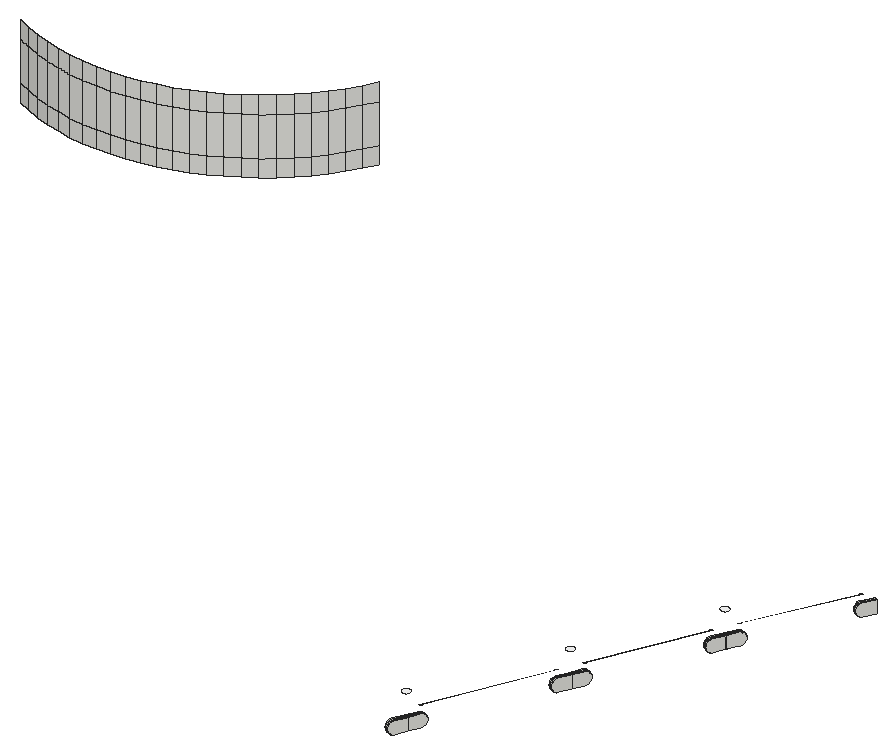
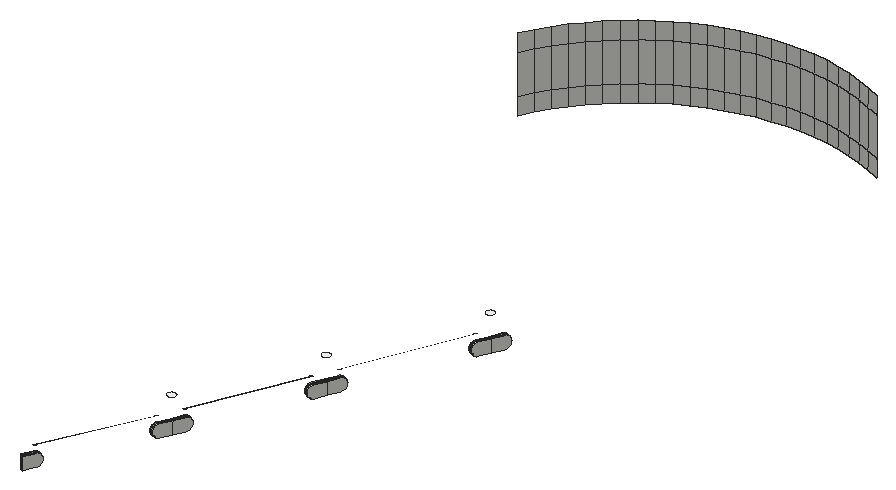
# SketchUp Ruby script. Lengths in inches.
U = 1.inch
M = Sketchup.active_model
def pt(a) = Geom::Point3d.new(a.map { |v| v * U })
def face(e, loops, mat)
  f = e.add_face(loops[0].map { |a| pt(a) })
  loops[1..].each { |l| e.add_face(l.map { |a| pt(a) }).erase! }
  f.material = f.back_material = mat if mat
  f
end
# faces: each face lists its corners as indices into pts; further lists are holes
def faces(e, pts, list, mat = nil) = list.each { |f| face(e, (f[0].is_a?(Array) ? f : [f]).map { |l| l.map { |i| pts[i] } }, mat) }
# xy, xz, yz: faces in a plane at the given z, y or x. An outline is a flat list of corners, or four numbers for a rectangle; further outlines are holes
def ring(l) = l.size == 4 ? [[l[0], l[1]], [l[2], l[1]], [l[2], l[3]], [l[0], l[3]]] : l.each_slice(2).to_a
def flat(e, list, mat, &to3) = list.each { |f| face(e, (f[0].is_a?(Array) ? f : [f]).map { |l| ring(l).map { |u, v| to3.(u, v) } }, mat) }
def xy(e, z, list, mat = nil) = flat(e, list, mat) { |x, y| [x, y, z] }
def xz(e, y, list, mat = nil) = flat(e, list, mat) { |x, z| [x, y, z] }
def yz(e, x, list, mat = nil) = flat(e, list, mat) { |y, z| [x, y, z] }
def lines(e, pts, list) = list.each { |a, b| e.add_line(pt(pts[a]), pt(pts[b])) }
# prism: a flat outline (further loops are holes) pulled along v
def prism(e, loops, v, mat = nil)
  f = face(e, loops, mat); d = Geom::Vector3d.new(v.map { |x| x * U })
  f.pushpull(f.normal.samedirection?(d) ? d.length : -d.length)
end
def box(e, o, s, mat = nil) = prism(e, [[o, [o[0] + s[0], o[1], o[2]], [o[0] + s[0], o[1] + s[1], o[2]], [o[0], o[1] + s[1], o[2]]]], [0, 0, s[2]], mat)
def at(x, y, z, deg = 0) = Geom::Transformation.translation(pt([x, y, z])) * Geom::Transformation.rotation(ORIGIN, Z_AXIS, deg.degrees)
def axes(o, x, y, z) = Geom::Transformation.new([*x, 0, *y, 0, *z, 0, *pt(o).to_a, 1])
def part(name) = M.definitions.add(name)
# library, detail: a bought-in or finely detailed component or shape, given as its bounding box
def library(name, o, s) = part(name).tap { |d| box(d.entities, o, s) }
def detail(e, o, s) = box(e.add_group.entities, o, s)
def put(e, d, t, mat = nil) = e.add_instance(d, t).tap { |i| i.material = mat if mat }
def group(e, t, mat = nil) = e.add_group.tap { |g| g.transformation = t; g.material = mat if mat }.entities
root = M.entities
M.materials.add("Glass_Safety_01").color = [204, 235, 244]
M.materials["Glass_Safety_01"].alpha = 0.1
M.materials.add("[Color_000]").color = [255, 255, 255]
xy(root,351.283,[[925.57,724.044,925.318,724.154,925.385,724.307,926.104,725.958,926.356,725.848],[925.137,724.232,924.884,724.342,925.67,726.147,925.923,726.037,925.204,724.386],[926.356,725.848,926.104,725.958,926.89,727.763,927.142,727.653],[925.923,726.037,925.67,726.147,926.456,727.952,926.709,727.842],[935.495,746.832,935.243,746.942,935.305,747.085,936.029,748.747,936.281,748.637],
  [935.062,747.021,934.809,747.131,935.595,748.935,935.848,748.825,935.124,747.164],[936.281,748.637,936.029,748.747,936.821,750.548,937.073,750.4375],[935.848,748.825,935.595,748.935,936.388,750.739,936.641,750.628],[944.885,768.202,944.633,768.313,944.699,768.465,945.424,770.112,945.673,769.993],[944.452,768.392,944.2,768.503,944.993,770.305,945.245,770.194,944.519,768.544],
  [945.673,769.993,945.424,770.112,945.425,770.115,945.677,770.004,945.675,769.999],[945.677,770.004,945.425,770.115,946.271,771.889,946.52,771.77],[945.246,770.197,944.997,770.315,945.844,772.092,946.093,771.974],[954.439,788.385,954.19,788.504,954.265,788.661,955.037,790.281,955.286,790.162],[954.013,788.589,953.764,788.707,954.6,790.46,954.857,790.359,954.087,788.745]])
xy(root,351.362,[[925.475,724.515,925.294,724.593,925.923,726.037,926.104,725.958],[926.104,725.958,925.923,726.037,926.552,727.481,926.732,727.402],[935.4,747.303,935.219,747.382,935.848,748.825,935.938,748.786,936.029,748.747],[936.029,748.747,935.938,748.786,935.848,748.825,936.482,750.267,936.662,750.188],[944.791,768.673,944.611,768.752,945.245,770.194,945.335,770.154,945.424,770.112],
  [945.424,770.112,945.335,770.154,945.425,770.115,945.424,770.113],[945.425,770.115,945.335,770.154,945.246,770.197,945.924,771.618,946.101,771.534]],"Glass_Safety_01")
xy(root,353.33,[[925.475,724.515,926.104,725.958,925.923,726.037,925.294,724.593],[926.104,725.958,926.732,727.402,926.552,727.481,925.923,726.037],[935.4,747.303,936.029,748.747,935.938,748.786,935.848,748.825,935.219,747.382],[936.029,748.747,936.662,750.188,936.482,750.267,935.848,748.825,935.938,748.786],[944.791,768.673,945.424,770.112,945.335,770.154,945.245,770.194,944.611,768.752],
  [945.424,770.112,945.424,770.113,945.425,770.115,945.335,770.154],[945.425,770.115,946.101,771.534,945.924,771.618,945.246,770.197,945.335,770.154]],"Glass_Safety_01")
xy(root,353.409,[[925.57,724.044,926.356,725.848,926.104,725.958,925.385,724.307,925.318,724.154],[925.137,724.232,925.204,724.386,925.923,726.037,925.67,726.147,924.884,724.342],[926.356,725.848,927.142,727.653,926.89,727.763,926.104,725.958],[925.923,726.037,926.709,727.842,926.456,727.952,925.67,726.147],[935.495,746.832,936.281,748.637,936.029,748.747,935.305,747.085,935.243,746.942],
  [935.062,747.021,935.124,747.164,935.848,748.825,935.595,748.935,934.809,747.131],[936.281,748.637,937.073,750.4375,936.821,750.548,936.029,748.747],[935.848,748.825,936.641,750.628,936.388,750.739,935.595,748.935],[944.885,768.202,945.673,769.993,945.424,770.112,944.699,768.465,944.633,768.313],[944.452,768.392,944.519,768.544,945.245,770.194,944.993,770.305,944.2,768.503],
  [945.673,769.993,945.675,769.999,945.677,770.004,945.425,770.115,945.424,770.112],[945.677,770.004,946.52,771.77,946.271,771.889,945.425,770.115],[945.246,770.197,946.093,771.974,945.844,772.092,944.997,770.315],[954.439,788.385,955.286,790.162,955.037,790.281,954.265,788.661,954.19,788.504],[954.013,788.589,954.087,788.745,954.857,790.359,954.6,790.46,953.764,788.707]])
xy(root,354.511,[[926.89,727.763,935.124,747.164,926.709,727.842],[926.89,727.763,935.305,747.085,935.124,747.164],[936.821,750.548,944.519,768.544,936.641,750.628],[936.821,750.548,944.7,768.465,944.519,768.544],[946.271,771.889,954.087,788.745,946.093,771.974],
  [946.271,771.889,954.265,788.661,954.087,788.745]],"Glass_Safety_01")
xy(root,357.267,[[926.058,725.369,926.219,725.402,926.367,725.476,926.489,725.585,926.58,725.723,926.632,725.879,926.642,726.043,926.609,726.204,926.535,726.351,926.426,726.474,926.289,726.564,926.132,726.616,925.968,726.626,925.807,726.593,925.66,726.519,925.537,726.41,925.447,726.273,925.395,726.117,925.385,725.953,925.418,725.792,925.492,725.645,925.601,725.522,925.738,725.431,925.894,725.379],[935.983,748.158,936.145,748.191,936.292,748.264,936.415,748.374,936.505,748.511,936.557,748.667,936.567,748.831,936.534,748.992,936.46,749.139,936.351,749.262,936.214,749.353,936.058,749.405,935.893,749.414,935.732,749.381,935.585,749.308,935.462,749.198,935.372,749.061,935.32,748.905,935.31,748.741,935.343,748.58,935.417,748.433,935.526,748.31,935.663,748.219,935.819,748.167],[945.38,769.526,945.541,769.559,945.688,769.633,945.811,769.742,945.902,769.879,945.954,770.035,945.963,770.199,945.93,770.361,945.857,770.508,945.747,770.631,945.61,770.721,945.454,770.773,945.29,770.783,945.129,770.75,944.982,770.676,944.859,770.567,944.768,770.43,944.716,770.274,944.707,770.109,944.74,769.948,944.813,769.801,944.923,769.678,945.06,769.588,945.216,769.536]],"[Color_000]")
p = [[926.356,725.848,353.409],[925.57,724.044,353.409],[925.46,723.791,353.373],[925.358,723.556,353.267],[925.27,723.354,353.098],[925.203,723.2,352.877],
  [925.16,723.102,352.621],[925.146,723.069,352.346],[925.16,723.102,352.071],[925.203,723.2,351.814],[925.27,723.354,351.594],[925.358,723.556,351.425],
  [925.46,723.791,351.319],[925.57,724.044,351.283],[926.356,725.848,351.283],[925.318,724.154,353.409],[925.385,724.307,353.409],[925.385,724.307,351.283],
  [925.318,724.154,351.283],[925.208,723.901,351.319],[925.105,723.666,351.425],[925.017,723.464,351.594],[924.95,723.31,351.814],[924.908,723.212,352.071],
  [924.893,723.179,352.346],[924.908,723.212,352.621],[924.95,723.31,352.877],[925.017,723.464,353.098],[925.105,723.666,353.267],[925.208,723.901,353.373],
  [925.137,724.232,351.283],[925.204,724.386,351.283],[925.204,724.386,353.409],[925.137,724.232,353.409],[925.027,723.98,353.373],[924.925,723.745,353.267],
  [924.837,723.543,353.098],[924.77,723.388,352.877],[924.727,723.291,352.621],[924.713,723.258,352.346],[924.727,723.291,352.071],[924.77,723.388,351.814],
  [924.837,723.543,351.594],[924.925,723.745,351.425],[925.027,723.98,351.319],[924.884,724.342,353.409],[925.67,726.147,353.409],[925.67,726.147,351.283],
  [924.884,724.342,351.283],[924.775,724.09,351.319],[924.672,723.855,351.425],[924.584,723.653,351.594],[924.517,723.498,351.814],[924.474,723.401,352.071],
  [924.46,723.368,352.346],[924.474,723.401,352.621],[924.517,723.498,352.877],[924.584,723.653,353.098],[924.672,723.855,353.267],[924.775,724.09,353.373],
  [926.104,725.958,351.283],[926.104,725.958,353.409],[926.104,725.958,353.33],[925.475,724.515,353.33],[925.475,724.515,351.362],[926.104,725.958,351.362],
  [925.923,726.037,353.409],[925.923,726.037,351.283],[925.923,726.037,351.362],[925.294,724.593,351.362],[925.294,724.593,353.33],[925.923,726.037,353.33],
  [927.142,727.653,353.409],[927.142,727.653,351.283],[927.252,727.905,351.319],[927.355,728.14,351.425],[927.442,728.342,351.594],[927.51,728.497,351.814],
  [927.552,728.594,352.071],[927.567,728.628,352.346],[927.552,728.594,352.621],[927.51,728.497,352.877],[927.442,728.342,353.098],[927.355,728.14,353.267],
  [927.252,727.905,353.373],[926.709,727.842,351.283],[926.709,727.842,353.409],[926.552,727.481,353.33],[926.552,727.481,351.362],[926.89,727.763,353.409],
  [926.89,727.763,351.283],[926.732,727.402,351.362],[926.732,727.402,353.33],[926.456,727.952,353.409],[926.566,728.204,353.373],[926.669,728.439,353.267],
  [926.757,728.641,353.098],[926.824,728.796,352.877],[926.866,728.893,352.621],[926.881,728.926,352.346],[926.866,728.893,352.071],[926.824,728.796,351.814],
  [926.757,728.641,351.594],[926.669,728.439,351.425],[926.566,728.204,351.319],[926.456,727.952,351.283],[926.999,728.015,351.319],[926.819,728.094,351.319],
  [926.819,728.094,353.373],[926.921,728.329,353.267],[927.009,728.531,353.098],[927.077,728.686,352.877],[927.119,728.783,352.621],[927.134,728.816,352.346],
  [927.119,728.783,352.071],[927.077,728.686,351.814],[927.009,728.531,351.594],[926.921,728.329,351.425],[927.102,728.25,351.425],[927.19,728.452,351.594],
  [927.257,728.607,351.814],[927.3,728.705,352.071],[927.314,728.738,352.346],[927.3,728.705,352.621],[927.257,728.607,352.877],[927.19,728.452,353.098],
  [927.102,728.25,353.267],[926.999,728.015,353.373],[936.281,748.637,353.409],[935.495,746.832,353.409],[935.385,746.58,353.373],[935.283,746.345,353.267],
  [935.195,746.143,353.098],[935.128,745.988,352.877],[935.085,745.891,352.621],[935.071,745.857,352.346],[935.085,745.891,352.071],[935.128,745.988,351.814],
  [935.195,746.143,351.594],[935.283,746.345,351.425],[935.385,746.58,351.319],[935.495,746.832,351.283],[936.281,748.637,351.283],[935.062,747.021,351.283],
  [935.124,747.164,351.283],[935.124,747.164,353.409],[935.062,747.021,353.409],[934.952,746.768,353.373],[934.85,746.533,353.267],[934.762,746.331,353.098],
  [934.695,746.177,352.877],[934.652,746.079,352.621],[934.638,746.046,352.346],[934.652,746.079,352.071],[934.695,746.177,351.814],[934.762,746.331,351.594],
  [934.85,746.533,351.425],[934.952,746.768,351.319],[935.243,746.942,353.409],[935.305,747.085,353.409],[935.305,747.085,351.283],[935.243,746.942,351.283],
  [935.133,746.69,351.319],[935.03,746.455,351.425],[934.942,746.253,351.594],[934.875,746.098,351.814],[934.833,746.001,352.071],[934.818,745.967,352.346],
  [934.833,746.001,352.621],[934.875,746.098,352.877],[934.942,746.253,353.098],[935.03,746.455,353.267],[935.133,746.69,353.373],[934.809,747.131,353.409],
  [935.595,748.935,353.409],[935.595,748.935,351.283],[934.809,747.131,351.283],[934.7,746.878,351.319],[934.597,746.643,351.425],[934.509,746.442,351.594],
  [934.442,746.287,351.814],[934.399,746.189,352.071],[934.385,746.156,352.346],[934.399,746.189,352.621],[934.442,746.287,352.877],[934.509,746.442,353.098],
  [934.597,746.643,353.267],[934.7,746.878,353.373],[936.029,748.747,351.283],[936.029,748.747,353.409],[936.029,748.747,353.33],[935.4,747.303,353.33],
  [935.4,747.303,351.362],[936.029,748.747,351.362],[935.848,748.825,353.409],[935.848,748.825,351.283],[935.848,748.825,351.362],[935.219,747.382,351.362],
  [935.219,747.382,353.33],[935.848,748.825,353.33],[937.073,750.4375,353.409],[937.073,750.4375,351.283],[937.184,750.689,351.319],[937.287,750.924,351.425],
  [937.376,751.126,351.594],[937.444,751.28,351.814],[937.486,751.377,352.071],[937.501,751.411,352.346],[937.486,751.377,352.621],[937.444,751.28,352.877],
  [937.376,751.126,353.098],[937.287,750.924,353.267],[937.184,750.689,353.373],[936.821,750.548,353.409],[936.821,750.548,351.283],[936.662,750.188,351.362],
  [936.662,750.188,353.33],[936.641,750.628,351.283],[936.641,750.628,353.409],[936.482,750.267,353.33],[936.482,750.267,351.362],[936.388,750.739,353.409],
  [936.499,750.99,353.373],[936.602,751.225,353.267],[936.691,751.427,353.098],[936.759,751.581,352.877],[936.802,751.678,352.621],[936.816,751.712,352.346],
  [936.802,751.678,352.071],[936.759,751.581,351.814],[936.691,751.427,351.594],[936.602,751.225,351.425],[936.499,750.99,351.319],[936.388,750.739,351.283],
  [936.932,750.8,351.319],[937.035,751.035,351.425],[937.123,751.236,351.594],[937.191,751.391,351.814],[937.234,751.488,352.071],[937.249,751.521,352.346],
  [937.234,751.488,352.621],[937.191,751.391,352.877],[937.123,751.236,353.098],[937.035,751.035,353.267],[936.932,750.8,353.373],[936.751,750.879,351.319],
  [936.751,750.879,353.373],[936.855,751.114,353.267],[936.943,751.316,353.098],[937.011,751.47,352.877],[937.054,751.568,352.621],[937.069,751.601,352.346],
  [937.054,751.568,352.071],[937.011,751.47,351.814],[936.943,751.316,351.594],[936.855,751.114,351.425],[944.885,768.202,351.283],[945.673,769.993,351.283],
  [945.673,769.993,353.409],[944.885,768.202,353.409],[944.774,767.95,353.373],[944.671,767.715,353.267],[944.582,767.514,353.098],[944.514,767.359,352.877],
  [944.472,767.262,352.621],[944.457,767.229,352.346],[944.472,767.262,352.071],[944.514,767.359,351.814],[944.582,767.514,351.594],[944.671,767.715,351.425],
  [944.774,767.95,351.319],[944.699,768.465,353.409],[945.424,770.112,353.409],[945.424,770.112,353.33],[945.424,770.112,351.362],[945.424,770.112,351.283],
  [944.699,768.465,351.283],[944.633,768.313,351.283],[944.522,768.061,351.319],[944.419,767.826,351.425],[944.33,767.625,351.594],[944.262,767.47,351.814],
  [944.219,767.373,352.071],[944.205,767.34,352.346],[944.219,767.373,352.621],[944.262,767.47,352.877],[944.33,767.625,353.098],[944.419,767.826,353.267],
  [944.522,768.061,353.373],[944.633,768.313,353.409],[944.452,768.392,351.283],[944.519,768.544,351.283],[944.519,768.544,353.409],[944.452,768.392,353.409],
  [944.342,768.14,353.373],[944.239,767.906,353.267],[944.15,767.704,353.098],[944.082,767.549,352.877],[944.039,767.452,352.621],[944.025,767.419,352.346],
  [944.039,767.452,352.071],[944.082,767.549,351.814],[944.15,767.704,351.594],[944.239,767.906,351.425],[944.342,768.14,351.319],[944.2,768.503,353.409],
  [944.993,770.305,353.409],[944.993,770.305,351.283],[944.2,768.503,351.283],[944.089,768.251,351.319],[943.986,768.016,351.425],[943.898,767.815,351.594],
  [943.83,767.66,351.814],[943.787,767.563,352.071],[943.772,767.53,352.346],[943.787,767.563,352.621],[943.83,767.66,352.877],[943.898,767.815,353.098],
  [943.986,768.016,353.267],[944.089,768.251,353.373],[945.245,770.194,353.409],[945.245,770.194,351.283],[945.245,770.194,351.362],[944.611,768.752,351.362],
  [944.611,768.752,353.33],[945.245,770.194,353.33],[945.425,770.115,351.283],[945.425,770.115,351.362],[945.425,770.115,353.33],[945.425,770.115,353.409],
  [945.677,770.004,353.409],[945.677,770.004,351.283],[945.675,769.999,353.409],[945.675,769.999,351.283],[946.52,771.77,351.283],[946.638,772.019,351.319],
  [946.748,772.25,351.425],[946.843,772.449,351.594],[946.916,772.601,351.814],[946.961,772.697,352.071],[946.977,772.73,352.346],[946.961,772.697,352.621],
  [946.916,772.601,352.877],[946.843,772.449,353.098],[946.748,772.25,353.267],[946.638,772.019,353.373],[946.52,771.77,353.409],[946.271,771.889,353.409],
  [946.389,772.137,353.373],[946.5,772.369,353.267],[946.594,772.568,353.098],[946.667,772.72,352.877],[946.713,772.816,352.621],[946.728,772.849,352.346],
  [946.713,772.816,352.071],[946.667,772.72,351.814],[946.594,772.568,351.594],[946.5,772.369,351.425],[946.389,772.137,351.319],[946.271,771.889,351.283],
  [945.246,770.197,351.283],[945.246,770.197,351.362],[945.246,770.197,353.33],[945.246,770.197,353.409],[944.997,770.315,353.409],[944.997,770.315,351.283],
  [946.093,771.974,351.283],[946.093,771.974,353.409],[945.924,771.618,353.33],[945.924,771.618,351.362],[945.844,772.092,353.409],[945.963,772.341,353.373],
  [946.073,772.572,353.267],[946.168,772.771,353.098],[946.24,772.923,352.877],[946.286,773.019,352.621],[946.302,773.052,352.346],[946.286,773.019,352.071],
  [946.24,772.923,351.814],[946.168,772.771,351.594],[946.073,772.572,351.425],[945.963,772.341,351.319],[945.844,772.092,351.283],[946.211,772.222,351.319],
  [946.211,772.222,353.373],[946.322,772.454,353.267],[946.417,772.652,353.098],[946.489,772.805,352.877],[946.535,772.901,352.621],[946.55,772.933,352.346],
  [946.535,772.901,352.071],[946.489,772.805,351.814],[946.417,772.652,351.594],[946.322,772.454,351.425],[955.286,790.162,353.409],[954.439,788.385,353.409],
  [954.321,788.137,353.373],[954.21,787.906,353.267],[954.116,787.707,353.098],[954.043,787.554,352.877],[953.997,787.459,352.621],[953.982,787.426,352.346],
  [953.997,787.459,352.071],[954.043,787.554,351.814],[954.116,787.707,351.594],[954.21,787.906,351.425],[954.321,788.137,351.319],[954.439,788.385,351.283],
  [955.286,790.162,351.283],[954.19,788.504,353.409],[954.265,788.661,353.409],[954.265,788.661,351.283],[954.19,788.504,351.283],[954.072,788.256,351.319],
  [953.962,788.024,351.425],[953.867,787.826,351.594],[953.794,787.673,351.814],[953.748,787.577,352.071],[953.733,787.544,352.346],[953.748,787.577,352.621],
  [953.794,787.673,352.877],[953.867,787.826,353.098],[953.962,788.024,353.267],[954.072,788.256,353.373],[954.013,788.589,351.283],[954.087,788.745,351.283],
  [954.857,790.359,351.283],[954.857,790.359,351.362],[954.857,790.359,353.33],[954.857,790.359,353.409],[954.087,788.745,353.409],[954.013,788.589,353.409],
  [953.894,788.34,353.373],[953.784,788.109,353.267],[953.689,787.91,353.098],[953.616,787.758,352.877],[953.571,787.662,352.621],[953.555,787.629,352.346],
  [953.571,787.662,352.071],[953.616,787.758,351.814],[953.689,787.91,351.594],[953.784,788.109,351.425],[953.894,788.34,351.319],[953.764,788.707,353.409],
  [954.6,790.46,353.409],[954.6,790.46,351.283],[953.764,788.707,351.283],[953.645,788.459,351.319],[953.535,788.228,351.425],[953.44,788.029,351.594],
  [953.368,787.876,351.814],[953.322,787.78,352.071],[953.306,787.748,352.346],[953.322,787.78,352.621],[953.368,787.876,352.877],[953.44,788.029,353.098],
  [953.535,788.228,353.267],[953.645,788.459,353.373],[955.037,790.281,351.283],[955.037,790.281,353.409],[955.037,790.281,353.33],[954.36,788.859,353.33],
  [954.36,788.859,351.362],[955.037,790.281,351.362],[935.938,748.786,351.362],[935.938,748.786,353.33],[944.791,768.673,351.362],[944.791,768.673,353.33],
  [945.335,770.154,353.33],[945.335,770.154,351.362],[945.424,770.113,351.362],[945.424,770.113,353.33],[946.101,771.534,353.33],[946.101,771.534,351.362],
  [954.182,788.944,353.33],[954.182,788.944,351.362],[860.46,738.588,415.758],[860.46,738.588,412.837],[862.815,738.526,412.837],[862.815,738.526,415.758],
  [865.169,738.617,412.837],[865.169,738.617,415.758],[858.115,738.805,415.758],[858.115,738.805,412.837],[867.512,738.862,412.837],[867.512,738.862,415.758],
  [855.788,739.175,415.758],[855.788,739.175,412.837],[869.834,739.26,412.837],[869.834,739.26,415.758],[853.491,739.695,415.758],[853.491,739.695,412.837],
  [872.125,739.809,412.837],[872.125,739.809,415.758],[851.232,740.366,415.758],[851.232,740.366,412.837],[874.375,740.507,412.837],[874.375,740.507,415.758],
  [849.022,741.182,415.758],[849.022,741.182,412.837],[876.575,741.35,412.837],[876.575,741.35,415.758],[846.871,742.141,415.758],[846.871,742.141,412.837],
  [878.715,742.336,412.837],[878.715,742.336,415.758],[880.786,743.459,412.837],[880.786,743.459,415.758],[882.779,744.715,412.837],[882.779,744.715,415.758],
  [884.685,746.099,412.837],[884.685,746.099,415.758],[886.497,747.604,412.837],[886.497,747.604,415.758],[888.206,749.225,412.837],[888.206,749.225,415.758],
  [889.806,750.954,412.837],[889.806,750.954,415.758],[891.29,752.785,412.837],[891.29,752.785,415.758],[892.65,754.708,412.837],[892.65,754.708,415.758],
  [893.882,756.716,412.837],[893.882,756.716,415.758],[894.98,758.8,412.837],[894.98,758.8,415.758],[862.815,738.526,422.51],[860.46,738.588,422.51],
  [865.169,738.617,422.51],[858.115,738.805,422.51],[867.512,738.862,422.51],[855.788,739.175,422.51],[869.834,739.26,422.51],[853.491,739.695,422.51],
  [872.125,739.809,422.51],[851.232,740.366,422.51],[874.375,740.507,422.51],[849.022,741.182,422.51],[876.575,741.35,422.51],[846.871,742.141,422.51],
  [878.715,742.336,422.51],[880.786,743.459,422.51],[882.779,744.715,422.51],[884.685,746.099,422.51],[886.497,747.604,422.51],[888.206,749.225,422.51],
  [889.806,750.954,422.51],[891.29,752.785,422.51],[892.65,754.708,422.51],[893.882,756.716,422.51],[894.98,758.8,422.51],[862.815,738.526,425.526],
  [860.46,738.588,425.526],[865.169,738.617,425.526],[858.115,738.805,425.526],[867.512,738.862,425.526],[855.788,739.175,425.526],[869.834,739.26,425.526],
  [853.491,739.695,425.526],[872.125,739.809,425.526],[851.232,740.366,425.526],[874.375,740.507,425.526],[849.022,741.182,425.526],[876.575,741.35,425.526],
  [846.871,742.141,425.526],[878.715,742.336,425.526],[880.786,743.459,425.526],[882.779,744.715,425.526],[884.685,746.099,425.526],[886.497,747.604,425.526],
  [888.206,749.225,425.526],[889.806,750.954,425.526],[891.29,752.785,425.526],[892.65,754.708,425.526],[893.882,756.716,425.526],[894.98,758.8,425.526]]
faces(root,p,[[0,1,2,3,4,5,6,7,8,9,10,11,12,13,14],[15,16,17,18,19,20,21,22,23,24,25,26,27,28,29],[30,31,32,33,34,35,36,37,38,39,40,41,42,43,44],[45,46,47,48,49,50,51,52,53,54,55,56,57,58,59],[20,19,12,11],[44,43,50,49],[19,18,13,12],[30,44,49,48],
  [60,17,16,61,62,63,64,65],[66,32,31,67,68,69,70,71],[60,65,62,61,0,14],[72,0,14,73,74,75,76,77,78,79,80,81,82,83,84],[68,67,47,46,66,71],[67,85,86,66,71,87,88,68],[61,89,90,60,65,91,92,62],[46,93,94,95,96,97,98,99,100,101,102,103,104,105,47],
  [90,106,74,73],[107,85,105,104],[106,118,75,74],[117,107,104,103],[128,129,130,131,132,133,134,135,136,137,138,139,140,141,142],[143,144,145,146,147,148,149,150,151,152,153,154,155,156,157],[158,159,160,161,162,163,164,165,166,167,168,169,170,171,172],[173,174,175,176,177,178,179,180,181,182,183,184,185,186,187],
  [163,162,140,139],[157,156,178,177],[162,161,141,140],[143,157,177,176],[188,160,159,189,190,191,192,193],[194,145,144,195,196,197,198,199],[188,193,190,189,128,142],[200,128,142,201,202,203,204,205,206,207,208,209,210,211,212],
  [189,213,214,188,193,215,216,190],[196,195,175,174,194,199],[195,217,218,194,199,219,220,196],[174,221,222,223,224,225,226,227,228,229,230,231,232,233,175],[214,234,202,201],[245,217,233,232],[234,235,203,202],[255,245,232,231],
  [256,257,258,259,260,261,262,263,264,265,266,267,268,269,270],[271,272,273,274,275,276,277,278,279,280,281,282,283,284,285,286,287,288,289],[290,291,292,293,294,295,296,297,298,299,300,301,302,303,304],[305,306,307,308,309,310,311,312,313,314,315,316,317,318,319],[279,278,270,269],[304,303,310,309],[278,277,256,270],[290,304,309,308],
  [320,292,291,321,322,323,324,325],[274,275,257,258,272,273],[326,327,328,329,330,331],[332,258,257,333,331,330],[332,258,257,333,331,334,335,336,337,338,339,340,341,342,343,344,345,346,330],[326,275,274,273,272,329,328,327],[272,329,347,348,349,350,351,352,353,354,355,356,357,358,359,326,275,274,273],[322,321,307,306,320,325],
  [360,361,362,363,364,365],[360,366,367,363,362,368,369,361],[364,370,371,372,373,374,375,376,377,378,379,380,381,382,365],[359,358,335,334],[383,366,382,381],[358,357,336,335],[393,383,381,380],[394,395,396,397,398,399,400,401,402,403,404,405,406,407,408],
  [409,410,411,412,413,414,415,416,417,418,419,420,421,422,423],[424,425,426,427,428,429,430,431,432,433,434,435,436,437,438,439,440,441,442],[443,444,445,446,447,448,449,450,451,452,453,454,455,456,457],[414,413,406,405],[442,441,448,447],[413,412,407,406],[424,442,447,446],[458,411,410,459,460,461,462,463],
  [21,20,11,10],[43,42,51,50],[118,119,76,75],[116,117,103,102],[164,163,139,138],[156,155,179,178],[235,236,204,203],[254,255,231,230],
  [280,279,269,268],[303,302,311,310],[357,356,337,336],[392,393,380,379],[415,414,405,404],[441,440,449,448],[22,21,10,9],[42,41,52,51],
  [119,120,77,76],[115,116,102,101],[165,164,138,137],[155,154,180,179],[236,237,205,204],[253,254,230,229],[281,280,268,267],[302,301,312,311],
  [356,355,338,337],[391,392,379,378],[416,415,404,403],[440,439,450,449],[41,40,53,52],[120,121,78,77],[114,115,101,100],[166,165,137,136],
  [154,153,181,180],[237,238,206,205],[252,253,229,228],[282,281,267,266],[301,300,313,312],[355,354,339,338],[390,391,378,377],[417,416,403,402],
  [439,438,451,450],[121,122,79,78],[113,114,100,99],[167,166,136,135],[153,152,182,181],[238,239,207,206],[251,252,228,227],[283,282,266,265],
  [300,299,314,313],[354,353,340,339],[389,390,377,376],[418,417,402,401],[438,437,452,451],[122,123,80,79],[112,113,99,98],[168,167,135,134],
  [152,151,183,182],[239,240,208,207],[250,251,227,226],[284,283,265,264],[299,298,315,314],[353,352,341,340],[388,389,376,375],[419,418,401,400],
  [437,436,453,452],[38,37,56,55],[123,124,81,80],[111,112,98,97],[169,168,134,133],[151,150,184,183],[240,241,209,208],[249,250,226,225],
  [285,284,264,263],[298,297,316,315],[352,351,342,341],[387,388,375,374],[420,419,400,399],[436,435,454,453],[27,26,5,4],[37,36,57,56],
  [124,125,82,81],[110,111,97,96],[170,169,133,132],[150,149,185,184],[241,242,210,209],[248,249,225,224],[286,285,263,262],[297,296,317,316],
  [351,350,343,342],[386,387,374,373],[421,420,399,398],[435,434,455,454],[28,27,4,3],[36,35,58,57],[125,126,83,82],[109,110,96,95],
  [171,170,132,131],[149,148,186,185],[242,243,211,210],[247,248,224,223],[287,286,262,261],[296,295,318,317],[350,349,344,343],[385,386,373,372],
  [422,421,398,397],[434,433,456,455],[29,28,3,2],[35,34,59,58],[126,127,84,83],[108,109,95,94],[172,171,131,130],[148,147,187,186],
  [243,244,212,211],[246,247,223,222],[288,287,261,260],[295,294,319,318],[349,348,345,344],[384,385,372,371],[423,422,397,396],[433,432,457,456],
  [15,29,2,1],[34,33,45,59],[127,89,72,84],[86,108,94,93],[158,172,130,129],[147,146,173,187],[244,213,200,212],[218,246,222,221],
  [289,288,260,259],[294,293,305,319],[348,347,346,345],[367,384,371,370],[409,423,396,395],[432,431,443,457],[476,477,478,479],[479,478,480,481],
  [482,483,477,476],[481,480,484,485],[486,487,483,482],[485,484,488,489],[490,491,487,486],[489,488,492,493],[494,495,491,490],[493,492,496,497],
  [498,499,495,494],[497,496,500,501],[502,503,499,498],[501,500,504,505],[505,504,506,507],[507,506,508,509],[509,508,510,511],[511,510,512,513],
  [513,512,514,515],[515,514,516,517],[517,516,518,519],[519,518,520,521],[521,520,522,523],[523,522,524,525],[476,479,526,527],[479,481,528,526],
  [482,476,527,529],[481,485,530,528],[486,482,529,531],[485,489,532,530],[490,486,531,533],[489,493,534,532],[494,490,533,535],[493,497,536,534],
  [498,494,535,537],[497,501,538,536],[502,498,537,539],[501,505,540,538],[505,507,541,540],[507,509,542,541],[509,511,543,542],[511,513,544,543],
  [513,515,545,544],[515,517,546,545],[517,519,547,546],[519,521,548,547],[521,523,549,548],[523,525,550,549],[527,526,551,552],[526,528,553,551],
  [529,527,552,554],[528,530,555,553],[531,529,554,556],[530,532,557,555],[533,531,556,558],[532,534,559,557],[535,533,558,560],[534,536,561,559],
  [537,535,560,562],[536,538,563,561],[539,537,562,564],[538,540,565,563],[540,541,566,565],[541,542,567,566],[542,543,568,567],[543,544,569,568],
  [544,545,570,569],[545,546,571,570],[546,547,572,571],[547,548,573,572],[548,549,574,573],[549,550,575,574]])
faces(root,p,[[85,86,108,109,110,111,112,113,114,115,116,117,107],[89,90,106,118,119,120,121,122,123,124,125,126,127],[213,214,234,235,236,237,238,239,240,241,242,243,244],[217,218,246,247,248,249,250,251,252,253,254,255,245],[347,359,358,357,356,355,354,353,352,351,350,349,348],[366,367,384,385,386,387,388,389,390,391,392,393,383],[70,69,64,63],[63,62,65,64],
  [71,70,69,68],[71,62,65,68],[87,71,68,88],[62,92,91,65],[92,91,88,87],[198,197,192,191],[191,190,193,192],[199,198,197,196],
  [193,464,465,190],[190,216,215,193],[199,465,464,196],[219,199,196,220],[219,216,215,220],[324,323,466,467],[466,274,273,467],[325,324,323,322],
  [468,469,274,273],[327,469,468,328],[470,327,328,471,273,274],[472,328,327,473],[325,468,469,322],[469,468,362,361],[368,362,361,369],[368,472,473,369],
  [474,475,462,461],[461,460,463,462]],"Glass_Safety_01")
